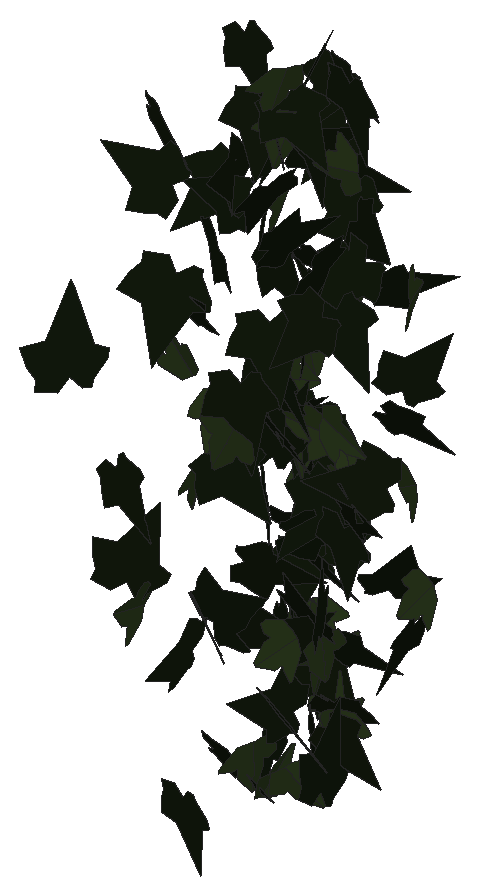
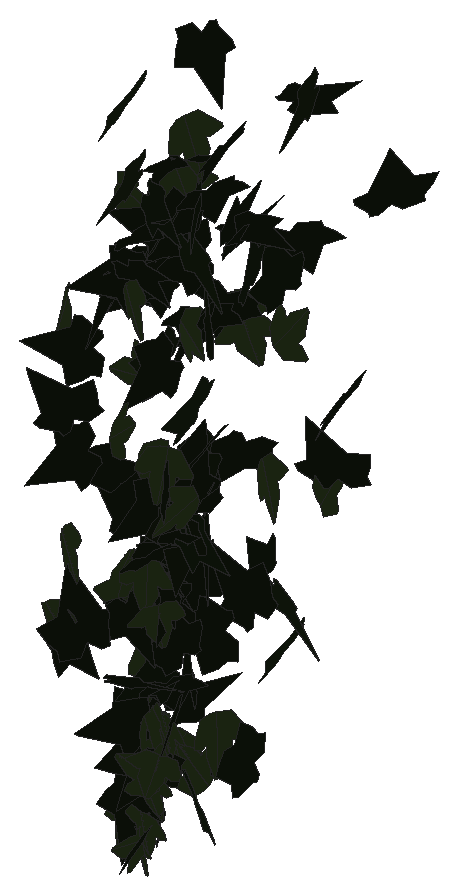
# SketchUp Ruby script. Lengths in inches.
U = 1.inch
M = Sketchup.active_model
def pt(a) = Geom::Point3d.new(a.map { |v| v * U })
def face(e, loops, mat)
  f = e.add_face(loops[0].map { |a| pt(a) })
  loops[1..].each { |l| e.add_face(l.map { |a| pt(a) }).erase! }
  f.material = f.back_material = mat if mat
  f
end
# faces: each face lists its corners as indices into pts; further lists are holes
def faces(e, pts, list, mat = nil) = list.each { |f| face(e, (f[0].is_a?(Array) ? f : [f]).map { |l| l.map { |i| pts[i] } }, mat) }
# xy, xz, yz: faces in a plane at the given z, y or x. An outline is a flat list of corners, or four numbers for a rectangle; further outlines are holes
def ring(l) = l.size == 4 ? [[l[0], l[1]], [l[2], l[1]], [l[2], l[3]], [l[0], l[3]]] : l.each_slice(2).to_a
def flat(e, list, mat, &to3) = list.each { |f| face(e, (f[0].is_a?(Array) ? f : [f]).map { |l| ring(l).map { |u, v| to3.(u, v) } }, mat) }
def xy(e, z, list, mat = nil) = flat(e, list, mat) { |x, y| [x, y, z] }
def xz(e, y, list, mat = nil) = flat(e, list, mat) { |x, z| [x, y, z] }
def yz(e, x, list, mat = nil) = flat(e, list, mat) { |y, z| [x, y, z] }
def lines(e, pts, list) = list.each { |a, b| e.add_line(pt(pts[a]), pt(pts[b])) }
# prism: a flat outline (further loops are holes) pulled along v
def prism(e, loops, v, mat = nil)
  f = face(e, loops, mat); d = Geom::Vector3d.new(v.map { |x| x * U })
  f.pushpull(f.normal.samedirection?(d) ? d.length : -d.length)
end
def box(e, o, s, mat = nil) = prism(e, [[o, [o[0] + s[0], o[1], o[2]], [o[0] + s[0], o[1] + s[1], o[2]], [o[0], o[1] + s[1], o[2]]]], [0, 0, s[2]], mat)
def at(x, y, z, deg = 0) = Geom::Transformation.translation(pt([x, y, z])) * Geom::Transformation.rotation(ORIGIN, Z_AXIS, deg.degrees)
def axes(o, x, y, z) = Geom::Transformation.new([*x, 0, *y, 0, *z, 0, *pt(o).to_a, 1])
def part(name) = M.definitions.add(name)
# library, detail: a bought-in or finely detailed component or shape, given as its bounding box
def library(name, o, s) = part(name).tap { |d| box(d.entities, o, s) }
def detail(e, o, s) = box(e.add_group.entities, o, s)
def put(e, d, t, mat = nil) = e.add_instance(d, t).tap { |i| i.material = mat if mat }
def group(e, t, mat = nil) = e.add_group.tap { |g| g.transformation = t; g.material = mat if mat }.entities
root = M.entities
M.materials.add("efeu1").color = [18, 25, 13]
M.materials.add("efeu2").color = [43, 57, 29]
c1 = part("ivyleaf_9")
p = [[1.54,2.16,1.25],[1.36,2.04,1.19],[-0.21,0.99,0.68],[-0.71,1.11,0.82],[-0.85,0.86,0.67],[-0.8,0.17,0.21],
  [-0.9,-0.01,0.1],[-0.67,-0.16,-0.02],[-0.08,-0.08,-0.05],[-0.03,-0.6,-0.4],[0.65,-0.88,-0.66],[0.83,-0.6,-0.49],
  [1.29,-0.42,-0.43],[1.8125,-0.07,-0.26],[1.21,0.44,0.15]]
faces(c1.entities,p,[[0,1,2,3,4,5,6,7,8,9,10,11,12,13,14]],"efeu1")
c2 = part("ivyleaf_10")
p = [[0,0.5,-0.03],[-0.0625,2.02,-0.43],[-0.19,2.01,-0.46],[-0.54,1.05,-0.29],[-0.52,0.625,-0.18],[-0.83,0.76,-0.28],
  [-1.16,0.64,-0.33],[-1.15,0.33,-0.24],[-0.77,-0.39,0.02],[-0.3,-0.51,0.16],[0.04,-0.48,0.23],[-0.02,2.01,-0.4375],
  [-0.06,2.01,-0.43],[0.04,-0.49,0.23],[0.67,-0.49,0.14],[1.38,0.36,-0.2],[1.375,0.51,-0.24],[0.81,0.65,-0.19],
  [0.62,0.59,-0.15],[0.6,1.09,-0.28],[0.5,1.23,-0.31]]
faces(c2.entities,p,[[0,1,2,3,4,5,6,7,8,9,10],[11,12,0,13,14,15,16,17,18,19,20]],"efeu2")
put(root,c1,axes([600.75,109.97,233.33],[-0.9515,-0.69548,0.84528],[0.68736,0.49202,1.17856],[-0.85189,1.17379,0.00681]))
put(root,c2,axes([601.14,114.67,219.22],[-0.1249,-0.39467,-1.17949],[-0.07967,-1.18045,0.40343],[-1.24121,0.11548,0.0928]))
put(root,c1,axes([603.51,114.8,209.9],[0.47593,-1.16558,0.30315],[0.11513,-0.28043,-1.259],[1.19884,0.48966,0.00056]))
put(root,c1,axes([600.4,114.65,220.49],[-0.92571,0.02936,0.96233],[0.95387,-0.15319,0.92224],[0.13065,1.32648,0.08521]))
put(root,c1,axes([599.46,115.14,225.48],[0.61287,-0.98298,-0.43993],[-0.2187,0.38203,-1.15829],[1.0545,0.65054,0.01546]))
put(root,c1,axes([601.84,115.87,240.99],[-0.75261,-0.8667,-0.49716],[-0.32753,-0.37403,1.14787],[-0.94396,0.82079,-0.0019]))
put(root,c2,axes([605.23,116.18,228.87],[-1.03628,-0.16877,0.63948],[-0.62006,-0.1656,-1.04852],[0.23009,-1.20639,0.05447]))
put(root,c1,axes([607.47,116.01,242.63],[-0.16299,1.13065,-0.45165],[0.07176,-0.44597,-1.14231],[-1.2154,-0.17795,-0.00687]))
put(root,c1,axes([600.76,117.625,234.96],[-0.84674,-1.13287,-0.29785],[0.20562,0.21806,-1.41395],[1.15318,-0.87071,0.03341]))
put(root,c1,axes([604.4,117.9,230.37],[-0.78208,-0.5897,-0.96526],[0.78091,0.56749,-0.97942],[0.81832,-1.10514,0.01213]))
put(root,c1,axes([606.26,117.85,214.51],[1.11023,-0.72334,0.32374],[0.27401,-0.17249,-1.32507],[0.74361,1.14353,0.00491]))
put(root,c2,axes([603.13,118.05,229.12],[0.88451,0.78328,-0.26797],[-0.19845,-0.1801,-1.18147],[-0.80371,0.9065,-0.00318]))
put(root,c1,axes([599.51,117.63,243.16],[0.94793,-0.38331,-0.6102],[-0.54819,0.27085,-1.02174],[0.46771,1.09433,0.03915]))
put(root,c1,axes([601.29,118.09,215.47],[-0.98026,0.91032,0.12526],[-0.09276,0.08419,-1.33775],[-0.9142,-0.98463,0.00142]))
put(root,c1,axes([600.21,118.89,232.79],[1.10355,-0.07825,-0.48047],[0.48007,-0.02228,1.10626],[-0.08064,-1.2034,0.01076]))
put(root,c1,axes([601.16,119.125,216.79],[0.71093,-0.19479,-1.06053],[1.04044,-0.2096,0.73596],[-0.2831,-1.25945,0.04154]))
put(root,c2,axes([600.41,118.75,229.79],[-0.92575,0.25651,-0.71186],[-0.6825,0.2026,0.96058],[0.32671,1.1501,-0.01044]))
put(root,c2,axes([606.05,119.11,217.13],[0.86412,-0.34512,-0.80747],[-0.76598,0.25775,-0.92987],[0.42941,1.15424,-0.03379]))
put(root,c1,axes([606.64,120.8125,233.48],[-0.65702,-0.8236,0.4983],[-0.27421,-0.41818,-1.05272],[0.92273,-0.7107,0.04197]))
put(root,c1,axes([607.88,119.23,218.37],[0.00849,0.13135,1.30354],[-0.19233,1.28957,-0.12869],[-1.29594,-0.19052,0.02763]))
put(root,c1,axes([600.74,120.66,215.78],[-0.11976,0.04414,1.44843],[1.11837,-0.92139,0.12055],[0.92149,1.12398,0.04194]))
put(root,c2,axes([599.875,120.64,223.55],[0.27457,-1.22543,-0.08057],[-0.01753,0.07864,-1.25581],[1.22795,0.27513,0.00009]))
put(root,c1,axes([601.375,120.44,224.43],[-0.01073,-0.71778,-1.04212],[0.20767,1.02703,-0.70952],[1.24824,-0.17704,0.10909]))
put(root,c1,axes([600.01,121.72,234.3125],[0.13407,-0.60939,1.16277],[0.22396,-1.14106,-0.62384],[1.29353,0.26072,-0.01251]))
put(root,c1,axes([603.8,120.67,215.47],[0.02269,-0.11814,1.26139],[1.26439,0.08161,-0.0151],[-0.07983,1.25895,0.11935]))
put(root,c1,axes([603.14,121.58,231.48],[-0.40316,-1.07731,-0.59291],[0.27962,0.5273,-1.14824],[1.19748,-0.48584,0.06851]))
put(root,c1,axes([605.21,121.78,216.88],[1.04834,-0.6352,0.39659],[-0.33556,0.21149,1.22575],[-0.66945,-1.10072,0.00666]))
put(root,c2,axes([602.24,121.44,209.17],[-0.37712,-1.18981,-0.14183],[0.04726,0.13381,-1.24813],[1.1973,-0.38004,0.00459]))
put(root,c1,axes([599.89,121.79,208.15],[0.9694,-0.51651,0.58443],[0.51099,-0.28379,-1.09838],[0.58927,1.0958,-0.00898]))
put(root,c1,axes([600.44,122.51,236.64],[0.13609,-1.07513,-0.30959],[0.04152,-0.3068,1.08371],[-1.11805,-0.14225,0.00256]))
put(root,c1,axes([606.44,121.17,208.8],[-0.27101,-0.59138,1.26391],[0.56956,1.12851,0.65016],[-1.27389,0.63038,0.0218]))
put(root,c1,axes([600.05,122.55,237.8],[-1.01715,-0.6559,0.31728],[-0.26774,-0.17025,-1.21029],[0.67764,-1.0518,-0.00195]))
put(root,c1,axes([606.8125,121.9,233.34],[0.14529,-1.13487,-0.69457],[-0.00534,0.6982,-1.14191],[1.33054,0.12673,0.07126]))
put(root,c2,axes([606.21,122.05,227.125],[0.20584,-0.10939,1.19448],[1.19898,0.05365,-0.2017],[-0.03453,1.2109,0.11685]))
put(root,c1,axes([600.08,123.33,237.39],[-0.0396,-0.2197,1.25326],[-0.35967,-1.20079,-0.22187],[1.22048,-0.361,-0.02472]))
put(root,c1,axes([603.01,123.25,210.68],[-0.23455,-0.15229,1.13008],[-0.89518,-0.69008,-0.27879],[0.70635,-0.92514,0.02194]))
put(root,c2,axes([603.86,122.37,208.1],[-0.85587,-0.53018,-0.63583],[0.52513,0.35932,-1.00648],[0.64,-1.00383,-0.02446]))
put(root,c2,axes([602.37,122.53,206.81],[0.0709,-1.03758,0.44217],[0.03402,0.44481,1.03831],[-1.12735,-0.05183,0.05914]))
put(root,c1,axes([602.73,122.21,235.12],[0.45918,0.52009,1.16295],[0.70729,0.92408,-0.69253],[-1.05957,0.84224,0.0417]))
put(root,c1,axes([601.58,123.875,227.79],[0.81097,-0.98195,0.20389],[0.12966,-0.15736,-1.27354],[0.99448,0.82127,-0.00023]))
put(root,c2,axes([601.96,124,243],[-0.35259,-1.17768,0.2315],[-0.10307,-0.21068,-1.22875],[1.19579,-0.36541,-0.03765]))
put(root,c1,axes([601.21,123.53,225.21],[1.24847,-0.12602,-0.34378],[-0.33425,0.10643,-1.25288],[0.14948,1.29056,0.06975]))
put(root,c1,axes([605.32,124.7,243.35],[0.47698,-1.23547,0.3499],[0.1119,-0.33185,-1.32426],[1.27917,0.48971,-0.01462]))
put(root,c1,axes([601.24,123.6,221.3125],[0.35644,-0.09156,-1.2622],[-1.2338,0.26658,-0.36776],[0.28153,1.28419,-0.01365]))
put(root,c1,axes([604.97,124.61,221.35],[0.45088,-0.42977,0.99442],[0.67814,-0.72801,-0.62211],[0.84482,0.81375,-0.03136]))
put(root,c2,axes([601.97,124.57,240.41],[-0.5977,-1.01434,0.36921],[-0.11457,-0.36003,-1.17461],[1.07335,-0.60327,0.08021]))
put(root,c1,axes([600.16,124.79,240.5625],[-0.35948,-1.15355,-0.18065],[0.06458,0.16908,-1.20822],[1.16583,-0.36506,0.01123]))
put(root,c1,axes([604.46,123.21,234.17],[-0.23649,0.46146,-1.19729],[-0.51077,1.08299,0.51829],[1.1771,0.56264,-0.01565]))
put(root,c1,axes([607.04,124.85,223.01],[-0.69924,-0.0748,1.06041],[-1.05648,-0.092,-0.70313],[0.118,-1.26686,-0.01155]))
put(root,c1,axes([601.875,124.51,241.44],[0.10077,-0.97999,-0.75342],[0.28699,0.75382,-0.94212],[1.20236,-0.09779,0.28802]))
put(root,c2,axes([603.83,124.49,213.9],[-0.40962,-1.06961,-0.20252],[0.0767,0.18749,-1.14535],[1.08591,-0.41671,0.0045]))
put(root,c1,axes([605.64,125.19,234.04],[-1.01202,-0.59753,0.14505],[-0.12527,-0.07311,-1.17526],[0.60199,-1.01975,-0.00073]))
put(root,c1,axes([600.96,125.06,214.33],[-0.18272,-0.08494,-1.09194],[1.08858,-0.13599,-0.17158],[-0.1206,-1.09874,0.10565]))
put(root,c1,axes([600.01,125.39,226.65],[0.37611,-1.26099,0.13977],[0.03557,-0.13524,-1.31587],[1.26821,0.37776,-0.00455]))
put(root,c1,axes([598.9375,125.04,243.62],[0.44778,-1.08533,-0.28321],[-0.12305,0.25557,-1.17396],[1.1149,0.46411,-0.01583]))
put(root,c1,axes([604.26,125.55,219.49],[0.19902,-1.14757,0.3867],[0.10738,-0.37362,-1.16402],[1.2062,0.22261,0.03982]))
put(root,c1,axes([600.76,124.64,233.29],[0.62246,-0.80782,-0.77802],[-0.4634,0.62507,-1.01975],[1.02135,0.77592,0.01149]))
put(root,c1,axes([601.24,125.25,224.18],[0.92758,0.02353,0.73982],[-0.73998,0.00048,0.92775],[0.01809,-1.18648,0.01505]))
put(root,c1,axes([599.53,124.49,216.625],[0.40711,0.39237,-1.14031],[0.73006,0.87774,0.56266],[0.95983,-0.83404,0.05569]))
put(root,c1,axes([601,124.55,240.03],[0.58009,-0.15207,-1.03385],[-0.99856,0.26783,-0.59968],[0.30797,1.15482,0.00294]))
put(root,c2,axes([603.49,124.97,224.57],[-0.0688,0.08761,-1.19349],[-1.1789,0.20046,0.08268],[0.20564,1.17855,0.07465]))
put(root,c2,axes([605.14,124.92,238.87],[-0.25013,0.05133,1.18971],[-1.18812,-0.09251,-0.2458],[0.08008,-1.2122,0.06914]))
put(root,c1,axes([600.96,124.62,222.8125],[-0.27719,-0.46797,1.12575],[0.87858,0.72371,0.51717],[-0.84522,0.90575,0.16841]))
put(root,c1,axes([599.24,125.75,232.92],[-0.02213,0.48515,1.08373],[0.06446,-1.08183,0.48561],[1.18562,0.06787,-0.00618]))
put(root,c1,axes([603.57,125.57,208.8],[0.02637,-0.25974,-1.18812],[1.04303,0.61599,-0.11152],[0.62545,-1.01631,0.23606]))
put(root,c1,axes([600.75,124.75,206.9],[-0.11109,0.57185,1.2489],[-0.40124,1.18482,-0.5782],[-1.31369,-0.41024,0.07099]))
put(root,c1,axes([601.67,126.44,238.32],[0.36999,-1.0058,0.46898],[0.14031,-0.44799,-1.07148],[1.10086,0.39514,-0.02106]))
put(root,c1,axes([600.41,125.77,237.91],[-0.7618,0.93038,-0.06435],[0.04916,-0.0429,-1.20243],[-0.93131,-0.76331,-0.01084]))
put(root,c1,axes([601.5625,126.46,231.49],[0.67062,-0.8364,0.47804],[0.34124,-0.33846,-1.0709],[0.90092,0.7508,0.04979]))
put(root,c1,axes([601.28,125.57,238.23],[0.34154,-0.01169,1.21299],[1.17928,0.29849,-0.32917],[-0.28425,1.2243,0.09184]))
put(root,c1,axes([602.43,126.65,220.23],[-1.2905,-0.23851,-0.15091],[0.14965,0.02066,-1.31234],[0.23931,-1.29913,0.00684]))
put(root,c1,axes([599.75,126.8,223.04],[-0.78414,0.48799,-0.73843],[0.44832,-0.63164,-0.89349],[-0.76316,-0.87246,0.23385]))
put(root,c1,axes([607.25,126.8125,214.91],[-0.49105,0.574,-0.91898],[0.53981,-0.74522,-0.75392],[-0.93947,-0.72822,0.04715]))
put(root,c1,axes([601.23,126.99,207.71],[-0.0265,-0.00046,-1.20975],[1.14362,-0.3946,-0.0249],[-0.3945,-1.14389,0.00907]))
put(root,c1,axes([601.13,125.76,218.16],[0.32664,0.66507,-0.97805],[0.35144,0.91426,0.73906],[1.12934,-0.47687,0.05289]))
put(root,c2,axes([600.1875,126.85,222.96],[-0.81187,0.46034,-0.71884],[0.44835,-0.61422,-0.89972],[-0.72638,-0.89364,0.2481]))
put(root,c2,axes([599.33,127.375,234.49],[0.42148,-0.93148,0.54692],[0.20976,-0.50532,-1.02229],[1.05961,0.47054,-0.01518]))
put(root,c1,axes([603.86,127.31,235.1],[-0.67975,-0.94569,-0.23585],[-0.12293,-0.20206,1.1645],[-0.96687,0.69054,0.01776]))
put(root,c2,axes([607.61,126.1875,232.46],[0.06112,-0.26829,-1.15406],[-0.26302,1.12369,-0.27516],[1.15527,0.27002,-0.00159]))
put(root,c2,axes([601.68,127.36,211.87],[0.22332,-1.12722,0.31047],[0.20802,-0.27274,-1.13984],[1.15054,0.2681,0.14582]))
put(root,c1,axes([604.42,126.46,235.21],[0.44882,-0.44443,-1.11754],[-0.80294,0.77732,-0.6316],[0.89539,0.91984,-0.00622]))
put(root,c1,axes([601.32,126.81,223.99],[1.1613,-0.09629,0.1445],[0.1425,-0.02989,-1.16514],[0.09922,1.16987,-0.01788]))
put(root,c1,axes([605.79,127.05,225.38],[1.13327,0.12166,0.35642],[0.35731,0.00994,-1.13946],[-0.11905,1.18795,-0.02697]))
put(root,c1,axes([600.77,127.09,232.08],[1.16151,0.09295,-0.04965],[-0.04962,-0.00236,-1.16522],[-0.09297,1.16257,0.00161]))
put(root,c1,axes([606.53,127.125,227.06],[-0.3756,-0.17962,1.12155],[1.12004,0.13775,0.39716],[-0.18877,1.17472,0.12492]))
put(root,c2,axes([600.35,127.72,212.92],[1.03512,-0.41985,0.20856],[0.19635,-0.07078,-1.117],[0.4257,1.05355,0.00807]))
put(root,c1,axes([599.36,127.77,217.08],[1.06034,0.19269,-0.25195],[0.24691,0.05044,1.0777],[0.19911,-1.0887,0.00533]))
put(root,c1,axes([599.99,127.05,223.23],[0.07983,1.17207,0.13639],[-0.04714,0.13976,-1.17344],[-1.17903,0.07377,0.05615]))
put(root,c2,axes([607.17,127.7,216.43],[0.90702,-0.41078,-0.67371],[-0.6179,0.26861,-0.99567],[0.49073,1.09746,-0.00848]))
put(root,c1,axes([605.0625,127.92,215.78],[1.1077,0.60197,0.32902],[-0.28889,-0.15746,1.2607],[0.62222,-1.14476,-0.00039]))
put(root,c1,axes([602.28,127.49,212.02],[0.93365,-0.02453,0.62165],[0.61991,-0.05792,-0.93333],[0.0525,1.12018,-0.03464]))
put(root,c1,axes([602.34,127.5,242],[0.92215,-0.49704,-0.47016],[-0.33928,0.35299,-1.03862],[0.59412,0.97304,0.13662]))
put(root,c1,axes([600.47,127.22,219.61],[-0.13986,0.12386,-1.10353],[-0.89553,0.64509,0.1859],[0.65662,0.90619,0.01849]))
put(root,c1,axes([599.65,128.43,215.43],[-0.48732,-0.958,-0.23688],[0.16484,0.18146,-1.07297],[0.97299,-0.51056,0.06313]))
put(root,c2,axes([600.28,127.93,227.29],[-1.06651,-0.36356,-0.07252],[0.075,0.0047,-1.12661],[0.36306,-1.06897,0.01971]))
put(root,c1,axes([600.13,128.625,223.06],[-0.55073,-0.99492,-0.04962],[0.0279,0.04127,-1.13717],[0.99577,-0.55142,0.00442]))
put(root,c1,axes([600.91,127.74,210.5],[-0.06018,-0.55867,-0.99023],[0.09697,0.98548,-0.56188],[1.13281,-0.11404,-0.00451]))
put(root,c1,axes([600.09,127.89,215.94],[1.12428,-0.23516,0.17058],[0.16597,-0.03968,-1.1486],[0.23844,1.13645,-0.00481]))
put(root,c2,axes([601.17,128.14,219.44],[0.04835,-0.0712,1.16573],[1.16209,0.11926,-0.04091],[-0.11644,1.16062,0.07572]))
put(root,c1,axes([599.61,127.72,213.98],[0.59207,-0.39384,-0.90621],[-0.7633,0.48855,-0.71103],[0.62745,0.96596,-0.00987]))
put(root,c1,axes([602.25,127.54,236.58],[0.166,0.36104,-1.12492],[0.54287,0.98563,0.39645],[1.04932,-0.56703,-0.02715]))
put(root,c2,axes([599.35,127.34,224.9],[-0.02247,0.4161,1.06815],[-0.0611,1.0664,-0.41671],[-1.14471,-0.06509,0.00128]))
put(root,c2,axes([601.64,128.39,206.59],[0.91496,-0.68472,-0.01362],[-0.00665,0.01384,-1.14278],[0.68483,0.91496,0.00709]))
put(root,c1,axes([605.0625,127.63,231.55],[0.3509,0.70583,-0.82974],[0.30391,0.77369,0.78667],[1.04609,-0.46153,0.04978]))
put(root,c2,axes([601.82,128.34,207.53],[-1.09887,-0.0535,-0.34198],[0.34605,-0.19472,-1.08151],[-0.00758,-1.13426,0.2018]))
put(root,c2,axes([600.9375,128.42,209.68],[1.03353,-0.12727,-0.25268],[-0.24424,0.08168,-1.04014],[0.1428,1.06083,0.04978]))
put(root,c1,axes([600.47,128.7,241.8],[-0.6817,0.54785,-0.70155],[0.5191,-0.47315,-0.87389],[-0.72308,-0.85616,0.03403]))
put(root,c1,axes([601.77,128.0625,208.52],[0.88393,0.61677,-0.46369],[-0.38976,-0.25166,-1.07773],[-0.66596,0.96592,0.0153]))
put(root,c1,axes([600.46,129.01,222.34],[-0.22697,-1.06971,-0.05845],[0.13872,0.0299,-1.08585],[1.06228,-0.23246,0.12931]))
put(root,c1,axes([602.12,128.4375,218.8],[0.26234,0.32968,-1.02575],[-0.94106,-0.44397,-0.38337],[-0.52465,0.96119,0.17475]))
put(root,c2,axes([600.89,128.62,221.34],[-1.11323,-0.18449,0.07523],[-0.0473,-0.17006,-1.11706],[0.19355,-1.10273,0.15969]))
put(root,c2,axes([602.4,128.54,219.72],[0.47818,1.09039,0.05461],[-0.03614,-0.04378,1.19053],[1.09116,-0.47929,0.0155]))
put(root,c1,axes([601.28,129.2,237.94],[-1.05166,-0.3726,-0.10365],[0.08965,0.05726,-1.11546],[0.37621,-1.0552,-0.02393]))
put(root,c1,axes([599.09,129.44,226.77],[-0.06967,-0.08333,-1.00986],[0.9105,-0.44938,-0.02573],[-0.44469,-0.90705,0.10552]))
put(root,c2,axes([600.5,128.46,210.0625],[-0.16286,-0.76671,0.793],[0.35035,0.72413,0.77208],[-1.04592,0.36195,0.13515]))
put(root,c2,axes([605.79,128.42,221.16],[0.5679,-0.30836,-0.97559],[-0.59832,0.80503,-0.60275],[0.82998,0.79133,0.23302]))
put(root,c1,axes([600.73,129.7,240.14],[-0.48809,-0.91359,0.347],[-0.03984,-0.36895,-1.02741],[0.97646,-0.47171,0.13154]))
put(root,c2,axes([599.72,129.01,219.6],[0.64576,0.90057,-0.11603],[-0.07546,-0.08866,-1.10813],[-0.90488,0.65008,0.0096]))
put(root,c2,axes([601.48,130.04,229.05],[0.02637,-0.19723,1.09826],[0.52669,-0.96628,-0.18617],[0.9837,0.52265,0.07024]))
put(root,c2,axes([601.29,129.16,236.4375],[0.66827,-0.3653,-0.84733],[-0.5388,0.69484,-0.7245],[0.74907,0.82569,0.23481]))
put(root,c1,axes([601.38,130.14,215.76],[-0.94248,0.08456,0.54988],[-0.54212,-0.38256,-0.87037],[0.12496,-1.0219,0.37133]))
put(root,c2,axes([600.01,129.81,208.54],[1.054,-0.14453,0.12272],[0.12004,-0.02787,-1.0638],[0.14677,1.06075,-0.01123]))
put(root,c2,axes([600.82,128.9,206.63],[0.22193,0.17867,-1.05559],[0.2894,1.02789,0.23482],[1.03075,-0.32707,0.16135]))
put(root,c2,axes([599.28,129.66,211.82],[0.87939,0.53234,0.32926],[0.23211,0.24999,-1.02408],[-0.58131,0.90512,0.08919]))
put(root,c1,axes([599.86,129.84,207.83],[0.54589,-0.83394,-0.35885],[-0.19476,0.3014,-0.99672],[0.88673,0.57959,0.002]))
